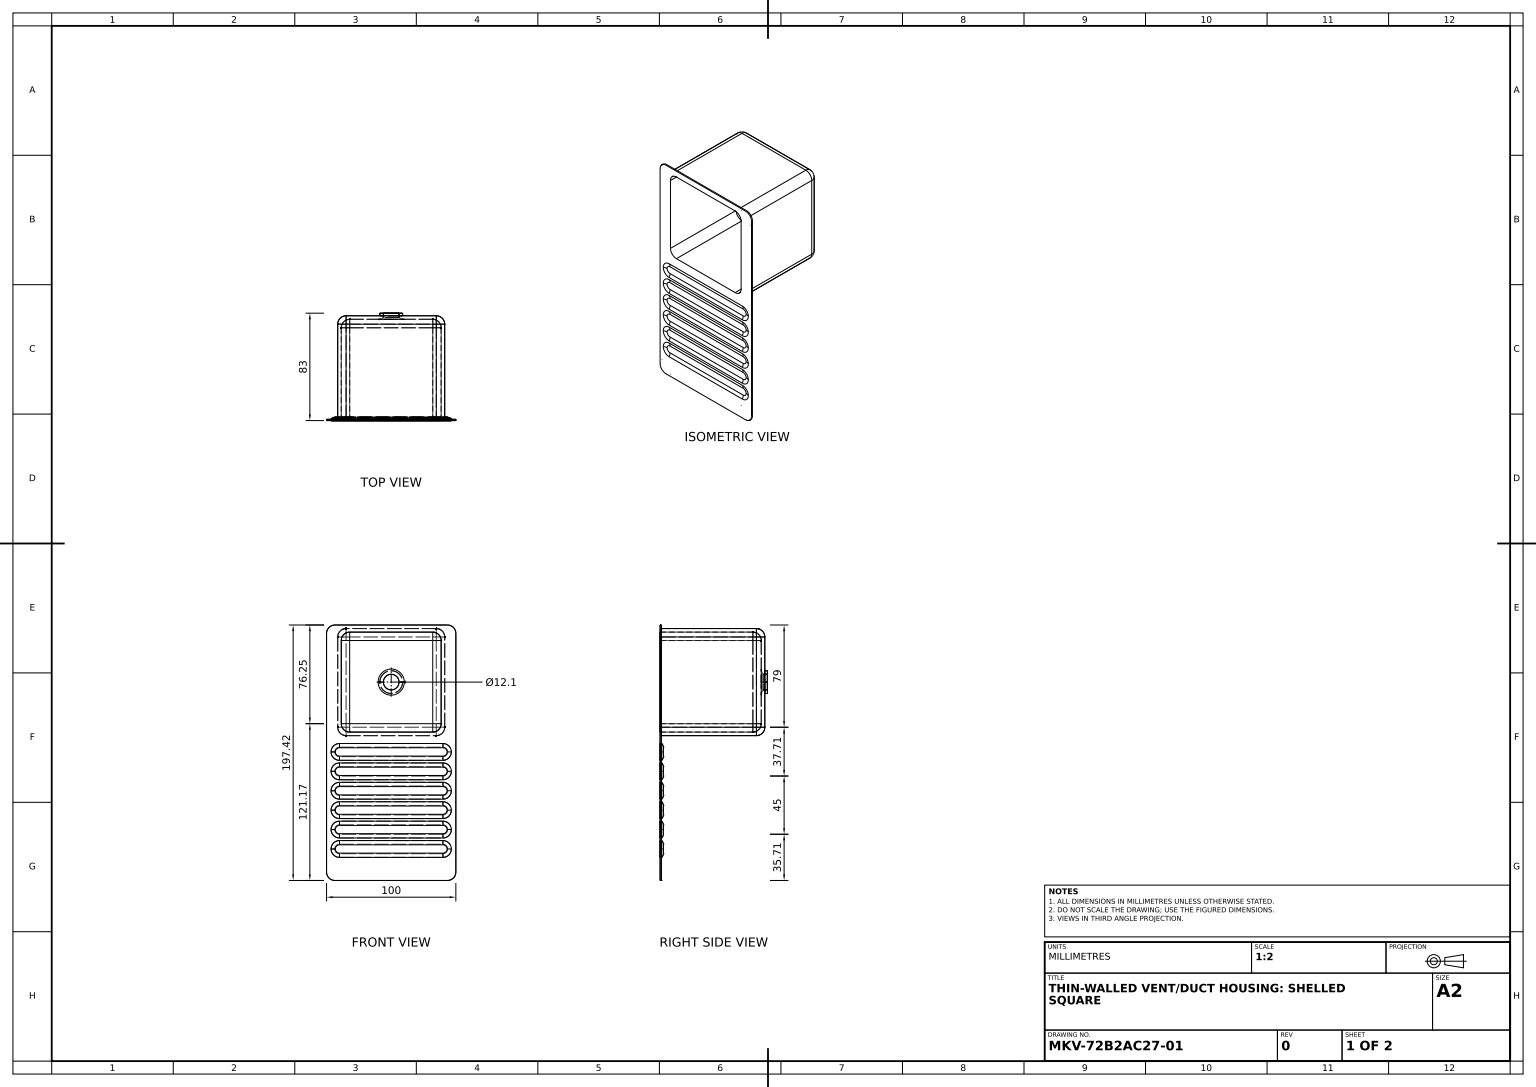
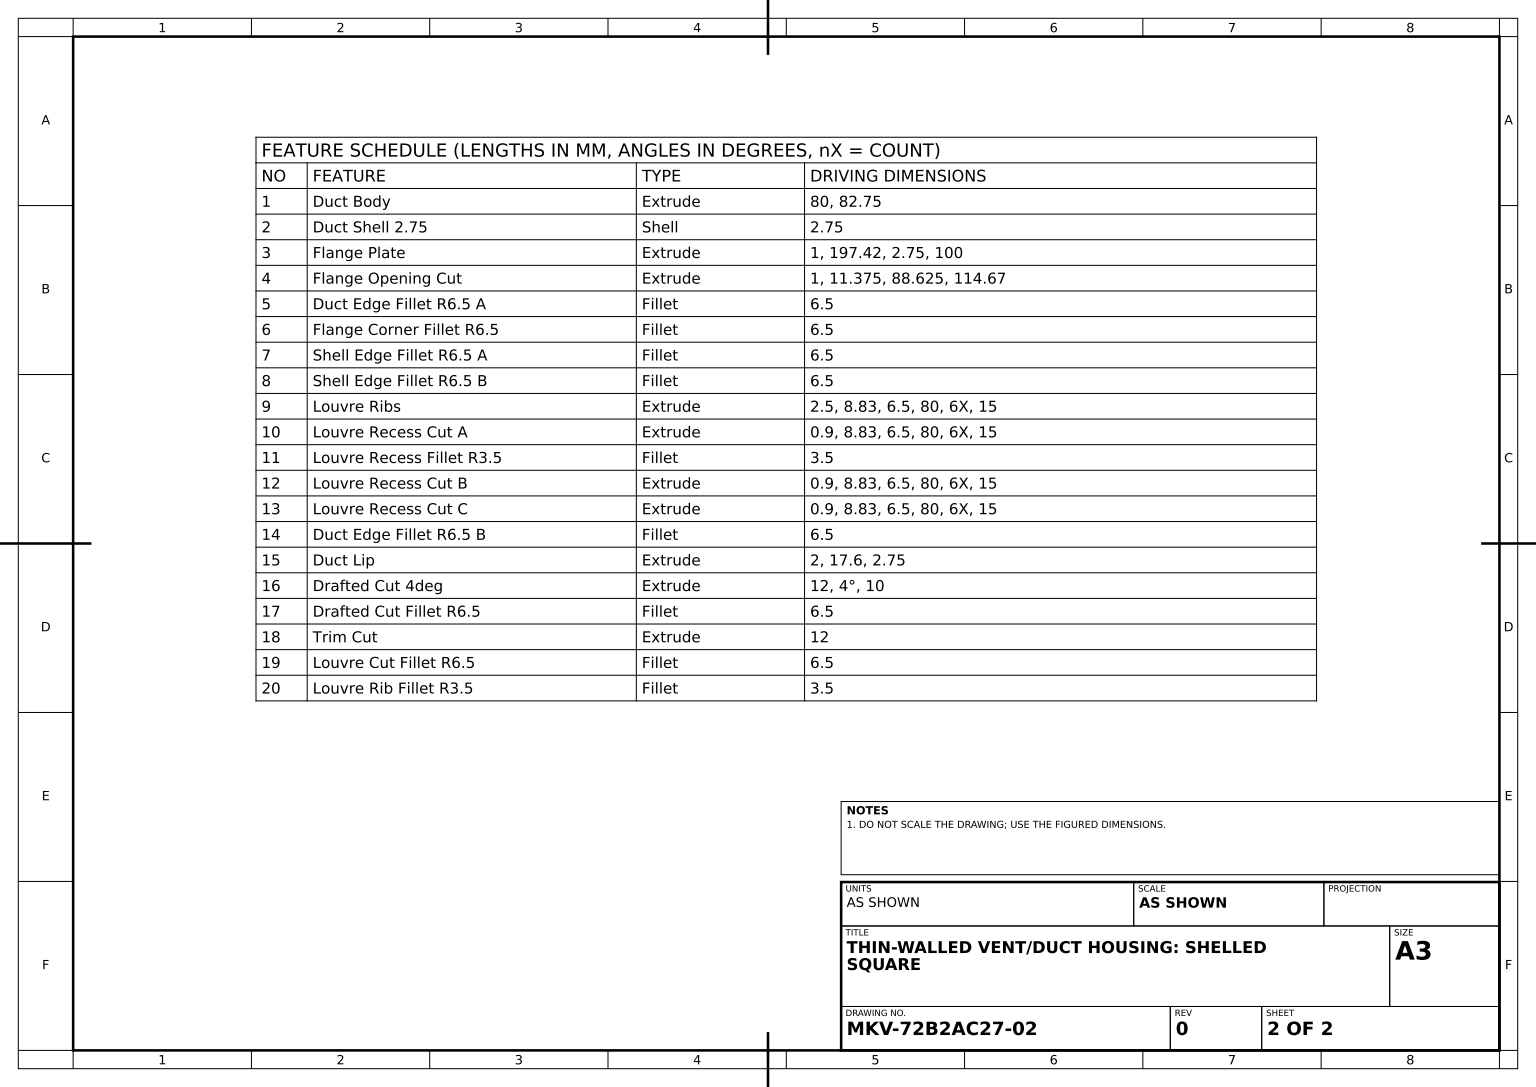
solid
v1 (40,-125.327281,38.5)
v2 (40,-132.582719,38.5)
e1 v1 v2 CIRCLE(AX(P(40,-128.955,38.5),D(0,0,-1),D(1,0,0)),3.627719)
v3 (-40,-132.582719,38.5)
e2 v2 v3 LINE
v4 (-43.627719,-128.955,38.5)
e3 v3 v4 CIRCLE(AX(P(-40,-128.955,38.5),D(0,0,-1),D(1,0,0)),3.627719)
v5 (-40,-125.327281,38.5)
e4 v4 v5 CIRCLE(AX(P(-40,-128.955,38.5),D(0,0,-1),D(1,0,0)),3.627719)
e5 v5 v1 LINE
face PLANE(AX(P(-40,-128.955,38.5),D(0,0,1),D(1,0,0))) rev [e1 e2 e3 e4 e5]
v6 (-40,-105.455,40)
v7 (40,-105.455,40)
e6 v6 v7 LINE
v8 (-40,-102.582719,38.5)
e7 v6 v8 CIRCLE(AX(P(-40,-102.582719,42),D(1,0,0),D(0,1,0)),3.5)
v9 (40,-102.582719,38.5)
e8 v9 v8 LINE
e9 v9 v7 CIRCLE(AX(P(40,-102.582719,42),D(-1,0,0),D(0,0,1)),3.5)
face CYL(AX(P(-40,-102.582719,42),D(-1,0,0),D(0,0,1)),3.5) [-e6 e7 -e8 e9]
v10 (-8.8,0,-42)
v11 (-8.8,0,-40)
e10 v10 v11 LINE
v12 (8.8,0,-42)
e11 v12 v10 CIRCLE(AX(P(0,0,-42),D(0,0,-1),D(-1,0,0)),8.8)
v13 (8.8,0,-40)
e12 v12 v13 LINE
e13 v13 v11 CIRCLE(AX(P(0,0,-40),D(0,0,-1),D(-1,0,0)),8.8)
face CYL(AX(P(0,0,-42),D(0,0,1),D(1,0,0)),8.8) [-e10 -e11 e12 e13]
v14 (-43.2,-53.955,40.1)
v15 (-40,-57.155,40.1)
e14 v14 v15 CIRCLE(AX(P(-40,-53.955,40.1),D(0,0,1),D(1,0,0)),3.2)
v16 (40,-57.155,40.1)
e15 v15 v16 LINE
v17 (43.2,-53.955,40.1)
e16 v16 v17 CIRCLE(AX(P(40,-53.955,40.1),D(0,0,1),D(1,0,0)),3.2)
v18 (40,-50.755,40.1)
e17 v17 v18 CIRCLE(AX(P(40,-53.955,40.1),D(0,0,1),D(1,0,0)),3.2)
v19 (-40,-50.755,40.1)
e18 v18 v19 LINE
e19 v19 v14 CIRCLE(AX(P(-40,-53.955,40.1),D(0,0,1),D(1,0,0)),3.2)
face PLANE(AX(P(-40,-53.955,40.1),D(0,0,1),D(1,0,0))) [e14 e15 e16 e17 e18 e19]
v20 (32.125,-32.125,-37.25)
v21 (32.125,32.125,-37.25)
e20 v20 v21 LINE
v22 (-32.125,32.125,-37.25)
e21 v21 v22 LINE
v23 (-32.125,-32.125,-37.25)
e22 v22 v23 LINE
e23 v23 v20 LINE
v24 (-10.116891,0,-37.25)
v25 (10.116891,0,-37.25)
e24 v24 v25 CIRCLE(AX(P(0,0,-37.25),D(0,0,-1),D(-1,0,0)),10.116891)
e25 v25 v24 CIRCLE(AX(P(0,0,-37.25),D(0,0,-1),D(-1,0,0)),10.116891)
face PLANE(AX(P(0,0,-37.25),D(0,0,-1),D(-1,0,0))) rev [e20 e21 e22 e23] [e24 e25]
v26 (-40,-122.455,40)
e26 v26 v5 CIRCLE(AX(P(-40,-125.327281,42),D(-1,0,0),D(0,0,1)),3.5)
v27 (40,-122.455,40)
e27 v27 v26 LINE
e28 v1 v27 CIRCLE(AX(P(40,-125.327281,42),D(1,0,0),D(0,0,-1)),3.5)
face CYL(AX(P(-40,-125.327281,42),D(1,0,0),D(0,1,0)),3.5) [-e5 -e26 -e27 -e28]
v28 (41.375,-34.875,-33.5)
v29 (41.375,34.875,-33.5)
e29 v28 v29 LINE
v30 (41.375,34.875,40)
e30 v29 v30 LINE
v31 (41.375,-34.875,40)
e31 v31 v30 LINE
e32 v31 v28 LINE
face PLANE(AX(P(41.375,-41.375,40),D(-1,0,0),D(0,0,1))) rev [e29 e30 -e31 e32]
v32 (40,-65.327281,38.5)
v33 (40,-72.582719,38.5)
e33 v32 v33 CIRCLE(AX(P(40,-68.955,38.5),D(0,0,-1),D(1,0,0)),3.627719)
v34 (-40,-72.582719,38.5)
e34 v33 v34 LINE
v35 (-43.627719,-68.955,38.5)
e35 v34 v35 CIRCLE(AX(P(-40,-68.955,38.5),D(0,0,-1),D(1,0,0)),3.627719)
v36 (-40,-65.327281,38.5)
e36 v35 v36 CIRCLE(AX(P(-40,-68.955,38.5),D(0,0,-1),D(1,0,0)),3.627719)
e37 v36 v32 LINE
face PLANE(AX(P(-40,-68.955,38.5),D(0,0,1),D(1,0,0))) rev [e33 e34 e35 e36 e37]
v37 (43.2,-68.955,40.1)
v38 (40,-65.755,40.1)
e38 v37 v38 CIRCLE(AX(P(40,-68.955,40.1),D(0,0,1),D(1,0,0)),3.2)
v39 (46.5,-68.955,41)
e39 v39 v37 CIRCLE(AX(P(43.2,-68.955,46.6),D(0,1,0),D(-1,0,0)),6.5)
v40 (40,-62.455,41)
e40 v39 v40 CIRCLE(AX(P(40,-68.955,41),D(0,0,1),D(1,0,0)),6.5)
e41 v38 v40 CIRCLE(AX(P(40,-65.755,46.6),D(1,0,0),D(0,0,-1)),6.5)
face TORUS(AX(P(40,-68.955,46.6),D(0,0,-1),D(-1,0,0)),3.2,6.5) rev [-e38 -e39 e40 -e41]
v41 (-38.625,32.125,-30.75)
v42 (-38.625,32.125,41)
e42 v41 v42 LINE
v43 (-32.125,38.625,-30.75)
e43 v41 v43 CIRCLE(AX(P(-32.125,32.125,-30.75),D(0,0,-1),D(1,0,0)),6.5)
v44 (-32.125,38.625,41)
e44 v44 v43 LINE
e45 v42 v44 CIRCLE(AX(P(-32.125,32.125,41),D(0,0,-1),D(1,0,0)),6.5)
face CYL(AX(P(-32.125,32.125,40),D(0,0,1),D(1,0,0)),6.5) rev [-e42 e43 -e44 -e45]
v45 (-6.05,0,-38.679458)
e46 v45 v24 CIRCLE(AX(P(-10.116891,0,-43.75),D(0,-1,0),D(0,0,-1)),6.5)
v46 (6.05,0,-38.679458)
e47 v46 v25 CIRCLE(AX(P(10.116891,0,-43.75),D(0,1,0),D(-1,0,0)),6.5)
e48 v45 v46 CIRCLE(AX(P(0,0,-38.679458),D(0,0,1),D(-1,0,0)),6.05)
face TORUS(AX(P(0,0,-43.75),D(0,0,-1),D(-1,0,0)),10.116891,6.5) [e46 -e25 -e47 -e48]
v47 (-46.5,-68.955,41)
v48 (-43.2,-68.955,40.1)
e49 v47 v48 CIRCLE(AX(P(-43.2,-68.955,46.6),D(0,-1,0),D(0,0,-1)),6.5)
v49 (-40,-75.455,41)
e50 v47 v49 CIRCLE(AX(P(-40,-68.955,41),D(0,0,1),D(1,0,0)),6.5)
v50 (-40,-72.155,40.1)
e51 v49 v50 CIRCLE(AX(P(-40,-72.155,46.6),D(1,0,0),D(0,0,-1)),6.5)
e52 v48 v50 CIRCLE(AX(P(-40,-68.955,40.1),D(0,0,1),D(1,0,0)),3.2)
face TORUS(AX(P(-40,-68.955,46.6),D(0,0,-1),D(-1,0,0)),3.2,6.5) rev [-e49 e50 e51 -e52]
v51 (-46.5,-113.955,40)
v52 (-43.627719,-113.955,38.5)
e53 v51 v52 CIRCLE(AX(P(-43.627719,-113.955,42),D(0,-1,0),D(0,0,-1)),3.5)
v53 (-40,-107.455,40)
e54 v53 v51 CIRCLE(AX(P(-40,-113.955,40),D(0,0,1),D(1,0,0)),6.5)
v54 (-40,-110.327281,38.5)
e55 v53 v54 CIRCLE(AX(P(-40,-110.327281,42),D(-1,0,0),D(0,0,1)),3.5)
e56 v52 v54 CIRCLE(AX(P(-40,-113.955,38.5),D(0,0,-1),D(1,0,0)),3.627719)
face TORUS(AX(P(-40,-113.955,42),D(0,0,-1),D(-1,0,0)),3.627719,3.5) [-e53 -e54 e55 -e56]
v55 (34.875,41.375,-33.5)
e57 v29 v55 CIRCLE(AX(P(34.875,34.875,-33.5),D(0,0,1),D(-1,0,0)),6.5)
v56 (34.875,41.375,40)
e58 v56 v55 LINE
e59 v30 v56 CIRCLE(AX(P(34.875,34.875,40),D(0,0,1),D(1,0,0)),6.5)
face CYL(AX(P(34.875,34.875,40),D(0,0,-1),D(-1,0,0)),6.5) [e57 -e58 -e59 -e30]
v57 (-40,-117.155,40.1)
v58 (40,-117.155,40.1)
e60 v57 v58 LINE
v59 (43.2,-113.955,40.1)
e61 v58 v59 CIRCLE(AX(P(40,-113.955,40.1),D(0,0,1),D(1,0,0)),3.2)
v60 (40,-110.755,40.1)
e62 v59 v60 CIRCLE(AX(P(40,-113.955,40.1),D(0,0,1),D(1,0,0)),3.2)
v61 (-40,-110.755,40.1)
e63 v60 v61 LINE
v62 (-43.2,-113.955,40.1)
e64 v61 v62 CIRCLE(AX(P(-40,-113.955,40.1),D(0,0,1),D(1,0,0)),3.2)
e65 v62 v57 CIRCLE(AX(P(-40,-113.955,40.1),D(0,0,1),D(1,0,0)),3.2)
face PLANE(AX(P(-40,-113.955,40.1),D(0,0,1),D(1,0,0))) [e60 e61 e62 e63 e64 e65]
v63 (40,-72.155,40.1)
e66 v63 v37 CIRCLE(AX(P(40,-68.955,40.1),D(0,0,1),D(1,0,0)),3.2)
v64 (40,-75.455,41)
e67 v63 v64 CIRCLE(AX(P(40,-72.155,46.6),D(-1,0,0),D(0,0,1)),6.5)
e68 v64 v39 CIRCLE(AX(P(40,-68.955,41),D(0,0,1),D(1,0,0)),6.5)
face TORUS(AX(P(40,-68.955,46.6),D(0,0,-1),D(-1,0,0)),3.2,6.5) rev [e39 -e66 e67 e68]
v65 (40,-135.455,40)
e69 v2 v65 CIRCLE(AX(P(40,-132.582719,42),D(-1,0,0),D(0,0,1)),3.5)
e70 v65 v27 CIRCLE(AX(P(40,-128.955,40),D(0,0,1),D(1,0,0)),6.5)
face TORUS(AX(P(40,-128.955,42),D(0,0,-1),D(-1,0,0)),3.627719,3.5) [-e69 -e1 e28 -e70]
v66 (-34.875,41.375,-33.5)
v67 (-34.875,34.875,-40)
e71 v66 v67 CIRCLE(AX(P(-34.875,34.875,-33.5),D(-1,0,0),D(0,0,1)),6.5)
v68 (-41.375,34.875,-33.5)
e72 v67 v68 CIRCLE(AX(P(-34.875,34.875,-33.5),D(0,1,0),D(0,0,1)),6.5)
e73 v66 v68 CIRCLE(AX(P(-34.875,34.875,-33.5),D(0,0,1),D(-1,0,0)),6.5)
face SPHERE(AX(P(-34.875,34.875,-33.5),D(0,1,0),D(-1,0,0)),6.5) [e71 e72 -e73]
v69 (40,-62.455,40)
e74 v32 v69 CIRCLE(AX(P(40,-65.327281,42),D(1,0,0),D(0,0,-1)),3.5)
v70 (40,-75.455,40)
e75 v70 v69 CIRCLE(AX(P(40,-68.955,40),D(0,0,1),D(1,0,0)),6.5)
e76 v33 v70 CIRCLE(AX(P(40,-72.582719,42),D(-1,0,0),D(0,0,1)),3.5)
face TORUS(AX(P(40,-68.955,42),D(0,0,-1),D(-1,0,0)),3.627719,3.5) [e74 -e75 -e76 -e33]
v71 (43.5,-153.295,41)
v72 (50,-146.795,41)
e77 v71 v72 CIRCLE(AX(P(43.5,-146.795,41),D(0,0,1),D(1,0,0)),6.5)
v73 (43.5,-153.295,40)
e78 v73 v71 LINE
v74 (50,-146.795,40)
e79 v74 v73 CIRCLE(AX(P(43.5,-146.795,40),D(0,0,-1),D(1,0,0)),6.5)
e80 v72 v74 LINE
face CYL(AX(P(43.5,-146.795,41),D(0,0,-1),D(-1,0,0)),6.5) [-e77 -e78 -e79 -e80]
v75 (40,-47.455,41)
e81 v18 v75 CIRCLE(AX(P(40,-50.755,46.6),D(1,0,0),D(0,0,-1)),6.5)
v76 (46.5,-53.955,41)
e82 v76 v17 CIRCLE(AX(P(43.2,-53.955,46.6),D(0,1,0),D(-1,0,0)),6.5)
e83 v76 v75 CIRCLE(AX(P(40,-53.955,41),D(0,0,1),D(1,0,0)),6.5)
face TORUS(AX(P(40,-53.955,46.6),D(0,0,-1),D(-1,0,0)),3.2,6.5) rev [-e81 -e17 -e82 e83]
e84 v11 v13 CIRCLE(AX(P(0,0,-40),D(0,0,-1),D(-1,0,0)),8.8)
e85 v10 v12 CIRCLE(AX(P(0,0,-42),D(0,0,-1),D(-1,0,0)),8.8)
face CYL(AX(P(0,0,-42),D(0,0,1),D(1,0,0)),8.8) [e84 -e12 -e85 e10]
v77 (-43.627719,-98.955,38.5)
v78 (-40,-95.327281,38.5)
e86 v77 v78 CIRCLE(AX(P(-40,-98.955,38.5),D(0,0,-1),D(1,0,0)),3.627719)
v79 (40,-95.327281,38.5)
e87 v78 v79 LINE
e88 v79 v9 CIRCLE(AX(P(40,-98.955,38.5),D(0,0,-1),D(1,0,0)),3.627719)
e89 v8 v77 CIRCLE(AX(P(-40,-98.955,38.5),D(0,0,-1),D(1,0,0)),3.627719)
face PLANE(AX(P(-40,-98.955,38.5),D(0,0,1),D(1,0,0))) rev [e86 e87 e88 e8 e89]
v80 (40,-87.155,40.1)
v81 (43.2,-83.955,40.1)
e90 v80 v81 CIRCLE(AX(P(40,-83.955,40.1),D(0,0,1),D(1,0,0)),3.2)
v82 (40,-90.455,41)
e91 v80 v82 CIRCLE(AX(P(40,-87.155,46.6),D(-1,0,0),D(0,0,1)),6.5)
v83 (46.5,-83.955,41)
e92 v82 v83 CIRCLE(AX(P(40,-83.955,41),D(0,0,1),D(1,0,0)),6.5)
e93 v83 v81 CIRCLE(AX(P(43.2,-83.955,46.6),D(0,1,0),D(-1,0,0)),6.5)
face TORUS(AX(P(40,-83.955,46.6),D(0,0,-1),D(-1,0,0)),3.2,6.5) rev [-e90 e91 e92 e93]
v84 (34.875,34.875,-40)
v85 (34.875,-34.875,-40)
e94 v84 v85 LINE
v86 (-34.875,-34.875,-40)
e95 v85 v86 LINE
e96 v86 v67 LINE
e97 v67 v84 LINE
face PLANE(AX(P(0,0,-40),D(0,0,-1),D(-1,0,0))) [-e84 -e13] [e94 e95 e96 e97]
v87 (-40,-105.455,41)
v88 (-40,-102.155,40.1)
e98 v87 v88 CIRCLE(AX(P(-40,-102.155,46.6),D(1,0,0),D(0,0,-1)),6.5)
v89 (-43.2,-98.955,40.1)
e99 v89 v88 CIRCLE(AX(P(-40,-98.955,40.1),D(0,0,1),D(1,0,0)),3.2)
v90 (-46.5,-98.955,41)
e100 v90 v89 CIRCLE(AX(P(-43.2,-98.955,46.6),D(0,-1,0),D(0,0,-1)),6.5)
e101 v90 v87 CIRCLE(AX(P(-40,-98.955,41),D(0,0,1),D(1,0,0)),6.5)
face TORUS(AX(P(-40,-98.955,46.6),D(0,0,-1),D(-1,0,0)),3.2,6.5) rev [e98 -e99 -e100 e101]
v91 (43.5,44.125,40)
v92 (50,37.625,40)
e102 v91 v92 CIRCLE(AX(P(43.5,37.625,40),D(0,0,-1),D(1,0,0)),6.5)
e103 v74 v92 LINE
v93 (-43.5,-153.295,40)
e104 v93 v73 LINE
v94 (-50,-146.795,40)
e105 v93 v94 CIRCLE(AX(P(-43.5,-146.795,40),D(0,0,-1),D(1,0,0)),6.5)
v95 (-50,37.625,40)
e106 v95 v94 LINE
v96 (-43.5,44.125,40)
e107 v95 v96 CIRCLE(AX(P(-43.5,37.625,40),D(0,0,-1),D(1,0,0)),6.5)
e108 v91 v96 LINE
v97 (-40,-60.455,40)
v98 (40,-60.455,40)
e109 v97 v98 LINE
v99 (40,-47.455,40)
e110 v98 v99 CIRCLE(AX(P(40,-53.955,40),D(0,0,1),D(1,0,0)),6.5)
v100 (-40,-47.455,40)
e111 v99 v100 LINE
v101 (-46.5,-53.955,40)
e112 v100 v101 CIRCLE(AX(P(-40,-53.955,40),D(0,0,1),D(1,0,0)),6.5)
e113 v101 v97 CIRCLE(AX(P(-40,-53.955,40),D(0,0,1),D(1,0,0)),6.5)
v102 (-46.5,-128.955,40)
e114 v26 v102 CIRCLE(AX(P(-40,-128.955,40),D(0,0,1),D(1,0,0)),6.5)
v103 (-40,-135.455,40)
e115 v102 v103 CIRCLE(AX(P(-40,-128.955,40),D(0,0,1),D(1,0,0)),6.5)
e116 v103 v65 LINE
v104 (40,-90.455,40)
v105 (40,-77.455,40)
e117 v104 v105 CIRCLE(AX(P(40,-83.955,40),D(0,0,1),D(1,0,0)),6.5)
v106 (-40,-77.455,40)
e118 v105 v106 LINE
v107 (-46.5,-83.955,40)
e119 v106 v107 CIRCLE(AX(P(-40,-83.955,40),D(0,0,1),D(1,0,0)),6.5)
v108 (-40,-90.455,40)
e120 v107 v108 CIRCLE(AX(P(-40,-83.955,40),D(0,0,1),D(1,0,0)),6.5)
e121 v108 v104 LINE
v109 (-40,-62.455,40)
e122 v69 v109 LINE
v110 (-46.5,-68.955,40)
e123 v109 v110 CIRCLE(AX(P(-40,-68.955,40),D(0,0,1),D(1,0,0)),6.5)
v111 (-40,-75.455,40)
e124 v110 v111 CIRCLE(AX(P(-40,-68.955,40),D(0,0,1),D(1,0,0)),6.5)
e125 v111 v70 LINE
v112 (40,-92.455,40)
v113 (-40,-92.455,40)
e126 v112 v113 LINE
v114 (-46.5,-98.955,40)
e127 v113 v114 CIRCLE(AX(P(-40,-98.955,40),D(0,0,1),D(1,0,0)),6.5)
e128 v114 v6 CIRCLE(AX(P(-40,-98.955,40),D(0,0,1),D(1,0,0)),6.5)
e129 v7 v112 CIRCLE(AX(P(40,-98.955,40),D(0,0,1),D(1,0,0)),6.5)
v115 (-41.375,-34.875,40)
v116 (-34.875,-41.375,40)
e130 v115 v116 CIRCLE(AX(P(-34.875,-34.875,40),D(0,0,1),D(1,0,0)),6.5)
v117 (34.875,-41.375,40)
e131 v116 v117 LINE
e132 v117 v31 CIRCLE(AX(P(34.875,-34.875,40),D(0,0,1),D(1,0,0)),6.5)
v118 (-34.875,41.375,40)
e133 v56 v118 LINE
v119 (-41.375,34.875,40)
e134 v118 v119 CIRCLE(AX(P(-34.875,34.875,40),D(0,0,1),D(1,0,0)),6.5)
e135 v119 v115 LINE
v120 (-40,-120.455,40)
v121 (40,-120.455,40)
e136 v120 v121 LINE
v122 (40,-107.455,40)
e137 v121 v122 CIRCLE(AX(P(40,-113.955,40),D(0,0,1),D(1,0,0)),6.5)
e138 v122 v53 LINE
e139 v51 v120 CIRCLE(AX(P(-40,-113.955,40),D(0,0,1),D(1,0,0)),6.5)
face PLANE(AX(P(0,0,40),D(0,0,1),D(1,0,0))) rev [e102 -e103 e79 -e104 e105 -e106 e107 -e108] [e109 e110 e111 e112 e113] [e27 e114 e115 e116 e70] [e117 e118 e119 e120 e121] [e75 e122 e123 e124 e125] [e126 e127 e128 e6 e129] [e130 e131 e132 e31 e59 e133 e134 e135] [e136 e137 e138 e54 e139]
v123 (-34.875,-41.375,-33.5)
v124 (34.875,-41.375,-33.5)
e140 v123 v124 LINE
e141 v124 v117 LINE
e142 v116 v123 LINE
face PLANE(AX(P(-41.375,-41.375,40),D(0,1,0),D(0,0,1))) rev [e140 e141 -e131 e142]
e143 v114 v77 CIRCLE(AX(P(-43.627719,-98.955,42),D(0,-1,0),D(0,0,-1)),3.5)
face TORUS(AX(P(-40,-98.955,42),D(0,0,-1),D(-1,0,0)),3.627719,3.5) [-e128 e143 -e89 -e7]
e144 v29 v84 CIRCLE(AX(P(34.875,34.875,-33.5),D(0,1,0),D(0,0,1)),6.5)
e145 v55 v84 CIRCLE(AX(P(34.875,34.875,-33.5),D(-1,0,0),D(0,0,1)),6.5)
face SPHERE(AX(P(34.875,34.875,-33.5),D(0,1,0),D(-1,0,0)),6.5) [e144 -e145 -e57]
v125 (-40,-50.327281,38.5)
v126 (40,-50.327281,38.5)
e146 v125 v126 LINE
e147 v100 v125 CIRCLE(AX(P(-40,-50.327281,42),D(-1,0,0),D(0,0,1)),3.5)
e148 v126 v99 CIRCLE(AX(P(40,-50.327281,42),D(1,0,0),D(0,0,-1)),3.5)
face CYL(AX(P(-40,-50.327281,42),D(1,0,0),D(0,1,0)),3.5) [-e146 -e147 -e111 -e148]
v127 (-40,-122.455,41)
v128 (-40,-125.755,40.1)
e149 v127 v128 CIRCLE(AX(P(-40,-125.755,46.6),D(-1,0,0),D(0,-1,0)),6.5)
v129 (-46.5,-128.955,41)
e150 v127 v129 CIRCLE(AX(P(-40,-128.955,41),D(0,0,1),D(1,0,0)),6.5)
v130 (-43.2,-128.955,40.1)
e151 v129 v130 CIRCLE(AX(P(-43.2,-128.955,46.6),D(0,-1,0),D(0,0,-1)),6.5)
e152 v128 v130 CIRCLE(AX(P(-40,-128.955,40.1),D(0,0,1),D(1,0,0)),3.2)
face TORUS(AX(P(-40,-128.955,46.6),D(0,0,-1),D(-1,0,0)),3.2,6.5) rev [-e149 e150 e151 -e152]
v131 (38.625,32.125,41)
v132 (38.625,32.125,-30.75)
e153 v131 v132 LINE
v133 (38.625,-32.125,-30.75)
e154 v132 v133 LINE
v134 (38.625,-32.125,41)
e155 v133 v134 LINE
e156 v134 v131 LINE
face PLANE(AX(P(38.625,-41.375,40),D(-1,0,0),D(0,0,1))) [e153 e154 e155 e156]
v135 (40,-135.455,41)
v136 (46.5,-128.955,41)
e157 v135 v136 CIRCLE(AX(P(40,-128.955,41),D(0,0,1),D(1,0,0)),6.5)
v137 (43.2,-128.955,40.1)
e158 v136 v137 CIRCLE(AX(P(43.2,-128.955,46.6),D(0,1,0),D(-1,0,0)),6.5)
v138 (40,-132.155,40.1)
e159 v138 v137 CIRCLE(AX(P(40,-128.955,40.1),D(0,0,1),D(1,0,0)),3.2)
e160 v138 v135 CIRCLE(AX(P(40,-132.155,46.6),D(-1,0,0),D(0,0,1)),6.5)
face TORUS(AX(P(40,-128.955,46.6),D(0,0,-1),D(-1,0,0)),3.2,6.5) rev [e157 e158 -e159 e160]
v139 (40,-77.455,41)
e161 v83 v139 CIRCLE(AX(P(40,-83.955,41),D(0,0,1),D(1,0,0)),6.5)
v140 (40,-80.755,40.1)
e162 v140 v139 CIRCLE(AX(P(40,-80.755,46.6),D(1,0,0),D(0,0,-1)),6.5)
e163 v81 v140 CIRCLE(AX(P(40,-83.955,40.1),D(0,0,1),D(1,0,0)),3.2)
face TORUS(AX(P(40,-83.955,46.6),D(0,0,-1),D(-1,0,0)),3.2,6.5) rev [e161 -e162 -e163 -e93]
v141 (40,-110.327281,38.5)
e164 v54 v141 LINE
v142 (40,-117.582719,38.5)
e165 v141 v142 CIRCLE(AX(P(40,-113.955,38.5),D(0,0,-1),D(1,0,0)),3.627719)
v143 (-40,-117.582719,38.5)
e166 v142 v143 LINE
e167 v143 v52 CIRCLE(AX(P(-40,-113.955,38.5),D(0,0,-1),D(1,0,0)),3.627719)
face PLANE(AX(P(-40,-113.955,38.5),D(0,0,1),D(1,0,0))) rev [e164 e165 e166 e167 e56]
e168 v46 v45 CIRCLE(AX(P(0,0,-38.679458),D(0,0,1),D(-1,0,0)),6.05)
face TORUS(AX(P(0,0,-43.75),D(0,0,-1),D(-1,0,0)),10.116891,6.5) [-e24 -e46 -e168 e47]
v144 (-32.125,-38.625,-30.75)
e169 v23 v144 CIRCLE(AX(P(-32.125,-32.125,-30.75),D(-1,0,0),D(0,0,1)),6.5)
v145 (32.125,-38.625,-30.75)
e170 v145 v144 LINE
e171 v20 v145 CIRCLE(AX(P(32.125,-32.125,-30.75),D(-1,0,0),D(0,0,1)),6.5)
face CYL(AX(P(0,-32.125,-30.75),D(1,0,0),D(0,0,-1)),6.5) rev [-e23 e169 -e170 -e171]
v146 (-40,-92.455,41)
e172 v146 v90 CIRCLE(AX(P(-40,-98.955,41),D(0,0,1),D(1,0,0)),6.5)
v147 (-40,-95.755,40.1)
e173 v147 v89 CIRCLE(AX(P(-40,-98.955,40.1),D(0,0,1),D(1,0,0)),3.2)
e174 v146 v147 CIRCLE(AX(P(-40,-95.755,46.6),D(-1,0,0),D(0,-1,0)),6.5)
face TORUS(AX(P(-40,-98.955,46.6),D(0,0,-1),D(-1,0,0)),3.2,6.5) rev [e172 e100 -e173 -e174]
v148 (-40,-62.455,41)
e175 v148 v40 LINE
v149 (-40,-65.755,40.1)
e176 v148 v149 CIRCLE(AX(P(-40,-65.755,46.6),D(-1,0,0),D(0,-1,0)),6.5)
e177 v38 v149 LINE
face CYL(AX(P(-40,-65.755,46.6),D(-1,0,0),D(0,-1,0)),6.5) rev [-e175 e176 -e177 e41]
v150 (40,-102.155,40.1)
v151 (40,-105.455,41)
e178 v150 v151 CIRCLE(AX(P(40,-102.155,46.6),D(-1,0,0),D(0,0,1)),6.5)
e179 v88 v150 LINE
e180 v87 v151 LINE
face CYL(AX(P(-40,-102.155,46.6),D(-1,0,0),D(0,0,1)),6.5) rev [-e178 -e179 -e98 e180]
v152 (-6.05,0,-42)
v153 (6.05,0,-42)
e181 v152 v153 CIRCLE(AX(P(0,0,-42),D(0,0,-1),D(-1,0,0)),6.05)
e182 v153 v152 CIRCLE(AX(P(0,0,-42),D(0,0,-1),D(-1,0,0)),6.05)
face PLANE(AX(P(0,0,-42),D(0,0,-1),D(-1,0,0))) [-e181 -e182] [e11 e85]
e183 v55 v66 LINE
e184 v66 v118 LINE
face PLANE(AX(P(-41.375,41.375,40),D(0,-1,0),D(0,0,-1))) rev [e183 e184 -e133 e58]
e185 v79 v112 CIRCLE(AX(P(40,-95.327281,42),D(1,0,0),D(0,0,-1)),3.5)
e186 v113 v78 CIRCLE(AX(P(-40,-95.327281,42),D(-1,0,0),D(0,0,1)),3.5)
face CYL(AX(P(-40,-95.327281,42),D(1,0,0),D(0,1,0)),3.5) [-e126 -e185 -e87 -e186]
v154 (40,-60.455,41)
e187 v16 v154 CIRCLE(AX(P(40,-57.155,46.6),D(-1,0,0),D(0,0,1)),6.5)
e188 v154 v76 CIRCLE(AX(P(40,-53.955,41),D(0,0,1),D(1,0,0)),6.5)
face TORUS(AX(P(40,-53.955,46.6),D(0,0,-1),D(-1,0,0)),3.2,6.5) rev [e187 e188 e82 -e16]
v155 (-40,-80.327281,38.5)
v156 (40,-80.327281,38.5)
e189 v155 v156 LINE
v157 (40,-87.582719,38.5)
e190 v156 v157 CIRCLE(AX(P(40,-83.955,38.5),D(0,0,-1),D(1,0,0)),3.627719)
v158 (-40,-87.582719,38.5)
e191 v157 v158 LINE
v159 (-43.627719,-83.955,38.5)
e192 v158 v159 CIRCLE(AX(P(-40,-83.955,38.5),D(0,0,-1),D(1,0,0)),3.627719)
e193 v159 v155 CIRCLE(AX(P(-40,-83.955,38.5),D(0,0,-1),D(1,0,0)),3.627719)
face PLANE(AX(P(-40,-83.955,38.5),D(0,0,1),D(1,0,0))) rev [e189 e190 e191 e192 e193]
e194 v120 v143 CIRCLE(AX(P(-40,-117.582719,42),D(1,0,0),D(0,1,0)),3.5)
face TORUS(AX(P(-40,-113.955,42),D(0,0,-1),D(-1,0,0)),3.627719,3.5) [-e194 -e139 e53 -e167]
v160 (-40,-47.455,41)
e195 v160 v19 CIRCLE(AX(P(-40,-50.755,46.6),D(-1,0,0),D(0,-1,0)),6.5)
v161 (-46.5,-53.955,41)
e196 v160 v161 CIRCLE(AX(P(-40,-53.955,41),D(0,0,1),D(1,0,0)),6.5)
e197 v161 v14 CIRCLE(AX(P(-43.2,-53.955,46.6),D(0,-1,0),D(0,0,-1)),6.5)
face TORUS(AX(P(-40,-53.955,46.6),D(0,0,-1),D(-1,0,0)),3.2,6.5) rev [-e195 e196 e197 -e19]
v162 (-41.375,-34.875,-33.5)
e198 v162 v123 CIRCLE(AX(P(-34.875,-34.875,-33.5),D(0,0,1),D(-1,0,0)),6.5)
e199 v86 v162 CIRCLE(AX(P(-34.875,-34.875,-33.5),D(0,1,0),D(0,0,1)),6.5)
e200 v86 v123 CIRCLE(AX(P(-34.875,-34.875,-33.5),D(-1,0,0),D(0,0,1)),6.5)
face SPHERE(AX(P(-34.875,-34.875,-33.5),D(0,1,0),D(-1,0,0)),6.5) [-e198 -e199 e200]
v163 (-40,-90.455,41)
v164 (-40,-87.155,40.1)
e201 v163 v164 CIRCLE(AX(P(-40,-87.155,46.6),D(1,0,0),D(0,0,-1)),6.5)
v165 (-43.2,-83.955,40.1)
e202 v165 v164 CIRCLE(AX(P(-40,-83.955,40.1),D(0,0,1),D(1,0,0)),3.2)
v166 (-46.5,-83.955,41)
e203 v166 v165 CIRCLE(AX(P(-43.2,-83.955,46.6),D(0,-1,0),D(0,0,-1)),6.5)
e204 v166 v163 CIRCLE(AX(P(-40,-83.955,41),D(0,0,1),D(1,0,0)),6.5)
face TORUS(AX(P(-40,-83.955,46.6),D(0,0,-1),D(-1,0,0)),3.2,6.5) rev [e201 -e202 -e203 e204]
v167 (-40,-120.455,41)
e205 v167 v57 CIRCLE(AX(P(-40,-117.155,46.6),D(1,0,0),D(0,0,-1)),6.5)
v168 (40,-120.455,41)
e206 v167 v168 LINE
e207 v58 v168 CIRCLE(AX(P(40,-117.155,46.6),D(-1,0,0),D(0,0,1)),6.5)
face CYL(AX(P(-40,-117.155,46.6),D(-1,0,0),D(0,-1,0)),6.5) rev [-e60 -e205 e206 -e207]
e208 v107 v159 CIRCLE(AX(P(-43.627719,-83.955,42),D(0,-1,0),D(0,0,-1)),3.5)
e209 v106 v155 CIRCLE(AX(P(-40,-80.327281,42),D(-1,0,0),D(0,0,1)),3.5)
face TORUS(AX(P(-40,-83.955,42),D(0,0,-1),D(-1,0,0)),3.627719,3.5) [-e193 -e208 -e119 e209]
v169 (-40,-77.455,41)
e210 v139 v169 LINE
v170 (-40,-80.755,40.1)
e211 v169 v170 CIRCLE(AX(P(-40,-80.755,46.6),D(-1,0,0),D(0,-1,0)),6.5)
e212 v140 v170 LINE
face CYL(AX(P(-40,-80.755,46.6),D(1,0,0),D(0,0,-1)),6.5) rev [e210 e211 -e212 e162]
v171 (40,-107.455,41)
e213 v60 v171 CIRCLE(AX(P(40,-110.755,46.6),D(1,0,0),D(0,0,-1)),6.5)
v172 (-40,-107.455,41)
e214 v171 v172 LINE
e215 v172 v61 CIRCLE(AX(P(-40,-110.755,46.6),D(-1,0,0),D(0,-1,0)),6.5)
face CYL(AX(P(-40,-110.755,46.6),D(1,0,0),D(0,0,-1)),6.5) rev [e213 e214 e215 -e63]
v173 (40,-125.755,40.1)
e216 v173 v128 LINE
v174 (40,-122.455,41)
e217 v173 v174 CIRCLE(AX(P(40,-125.755,46.6),D(1,0,0),D(0,0,-1)),6.5)
e218 v174 v127 LINE
face CYL(AX(P(-40,-125.755,46.6),D(1,0,0),D(0,1,0)),6.5) rev [e149 -e216 e217 e218]
v175 (-43.627719,-53.955,38.5)
e219 v175 v125 CIRCLE(AX(P(-40,-53.955,38.5),D(0,0,-1),D(1,0,0)),3.627719)
e220 v101 v175 CIRCLE(AX(P(-43.627719,-53.955,42),D(0,-1,0),D(0,0,-1)),3.5)
face TORUS(AX(P(-40,-53.955,42),D(0,0,-1),D(-1,0,0)),3.627719,3.5) [-e112 e147 -e219 -e220]
v176 (-40,-60.455,41)
e221 v176 v15 CIRCLE(AX(P(-40,-57.155,46.6),D(1,0,0),D(0,0,-1)),6.5)
e222 v161 v176 CIRCLE(AX(P(-40,-53.955,41),D(0,0,1),D(1,0,0)),6.5)
face TORUS(AX(P(-40,-53.955,46.6),D(0,0,-1),D(-1,0,0)),3.2,6.5) rev [e221 -e14 -e197 e222]
v177 (-38.625,-32.125,-30.75)
e223 v144 v177 CIRCLE(AX(P(-32.125,-32.125,-30.75),D(0,0,-1),D(1,0,0)),6.5)
e224 v23 v177 CIRCLE(AX(P(-32.125,-32.125,-30.75),D(0,1,0),D(0,0,1)),6.5)
face SPHERE(AX(P(-32.125,-32.125,-30.75),D(0,1,0),D(-1,0,0)),6.5) rev [-e223 -e169 e224]
e225 v85 v124 CIRCLE(AX(P(34.875,-34.875,-33.5),D(-1,0,0),D(0,-1,0)),6.5)
face CYL(AX(P(-41.375,-34.875,-33.5),D(-1,0,0),D(0,0,1)),6.5) [-e200 -e95 e225 -e140]
e226 v111 v34 CIRCLE(AX(P(-40,-72.582719,42),D(1,0,0),D(0,1,0)),3.5)
face CYL(AX(P(-40,-72.582719,42),D(-1,0,0),D(0,0,1)),3.5) [-e34 e76 -e125 e226]
e227 v149 v48 CIRCLE(AX(P(-40,-68.955,40.1),D(0,0,1),D(1,0,0)),3.2)
e228 v50 v63 LINE
face PLANE(AX(P(-40,-68.955,40.1),D(0,0,1),D(1,0,0))) [e177 e227 e52 e228 e66 e38]
v178 (32.125,38.625,41)
e229 v178 v44 LINE
v179 (32.125,38.625,-30.75)
e230 v43 v179 LINE
e231 v179 v178 LINE
face PLANE(AX(P(-41.375,38.625,40),D(0,-1,0),D(0,0,-1))) [e229 e44 e230 e231]
v180 (-40,-132.155,40.1)
e232 v180 v138 LINE
v181 (-40,-135.455,41)
e233 v181 v180 CIRCLE(AX(P(-40,-132.155,46.6),D(1,0,0),D(0,0,-1)),6.5)
e234 v181 v135 LINE
face CYL(AX(P(-40,-132.155,46.6),D(-1,0,0),D(0,0,1)),6.5) rev [-e160 -e232 -e233 e234]
v182 (-40,-57.582719,38.5)
e235 v182 v175 CIRCLE(AX(P(-40,-53.955,38.5),D(0,0,-1),D(1,0,0)),3.627719)
e236 v97 v182 CIRCLE(AX(P(-40,-57.582719,42),D(1,0,0),D(0,1,0)),3.5)
face TORUS(AX(P(-40,-53.955,42),D(0,0,-1),D(-1,0,0)),3.627719,3.5) [-e113 e220 -e235 -e236]
e237 v68 v162 LINE
e238 v162 v115 LINE
e239 v119 v68 LINE
face PLANE(AX(P(-41.375,-41.375,40),D(1,0,0),D(0,0,-1))) rev [e237 e238 -e135 e239]
e240 v22 v41 CIRCLE(AX(P(-32.125,32.125,-30.75),D(0,1,0),D(0,0,1)),6.5)
e241 v177 v41 LINE
face CYL(AX(P(-32.125,0,-30.75),D(0,-1,0),D(0,0,-1)),6.5) rev [-e22 e240 -e241 -e224]
e242 v133 v145 CIRCLE(AX(P(32.125,-32.125,-30.75),D(0,0,-1),D(1,0,0)),6.5)
v183 (32.125,-38.625,41)
e243 v183 v145 LINE
e244 v134 v183 CIRCLE(AX(P(32.125,-32.125,41),D(0,0,-1),D(1,0,0)),6.5)
face CYL(AX(P(32.125,-32.125,40),D(0,0,1),D(1,0,0)),6.5) rev [-e155 e242 -e243 -e244]
face CYL(AX(P(-34.875,-34.875,40),D(0,0,-1),D(-1,0,0)),6.5) [-e238 e198 -e142 -e130]
e245 v148 v47 CIRCLE(AX(P(-40,-68.955,41),D(0,0,1),D(1,0,0)),6.5)
face TORUS(AX(P(-40,-68.955,46.6),D(0,0,-1),D(-1,0,0)),3.2,6.5) rev [-e227 -e176 e245 e49]
e246 v109 v36 CIRCLE(AX(P(-40,-65.327281,42),D(-1,0,0),D(0,0,1)),3.5)
e247 v110 v35 CIRCLE(AX(P(-43.627719,-68.955,42),D(0,-1,0),D(0,0,-1)),3.5)
face TORUS(AX(P(-40,-68.955,42),D(0,0,-1),D(-1,0,0)),3.627719,3.5) [-e123 e246 -e36 -e247]
e248 v179 v21 CIRCLE(AX(P(32.125,32.125,-30.75),D(-1,0,0),D(0,0,1)),6.5)
e249 v43 v22 CIRCLE(AX(P(-32.125,32.125,-30.75),D(-1,0,0),D(0,0,1)),6.5)
face CYL(AX(P(0,32.125,-30.75),D(-1,0,0),D(0,0,1)),6.5) rev [-e21 -e248 -e230 e249]
v184 (40,-92.455,41)
e250 v184 v146 LINE
v185 (46.5,-98.955,41)
e251 v185 v184 CIRCLE(AX(P(40,-98.955,41),D(0,0,1),D(1,0,0)),6.5)
e252 v151 v185 CIRCLE(AX(P(40,-98.955,41),D(0,0,1),D(1,0,0)),6.5)
e253 v136 v174 CIRCLE(AX(P(40,-128.955,41),D(0,0,1),D(1,0,0)),6.5)
e254 v129 v181 CIRCLE(AX(P(-40,-128.955,41),D(0,0,1),D(1,0,0)),6.5)
e255 v176 v154 LINE
e256 v160 v75 LINE
e257 v49 v64 LINE
v186 (46.5,-113.955,41)
e258 v168 v186 CIRCLE(AX(P(40,-113.955,41),D(0,0,1),D(1,0,0)),6.5)
v187 (-46.5,-113.955,41)
e259 v187 v167 CIRCLE(AX(P(-40,-113.955,41),D(0,0,1),D(1,0,0)),6.5)
e260 v172 v187 CIRCLE(AX(P(-40,-113.955,41),D(0,0,1),D(1,0,0)),6.5)
e261 v186 v171 CIRCLE(AX(P(40,-113.955,41),D(0,0,1),D(1,0,0)),6.5)
e262 v169 v166 CIRCLE(AX(P(-40,-83.955,41),D(0,0,1),D(1,0,0)),6.5)
e263 v163 v82 LINE
v188 (-32.125,-38.625,41)
e264 v188 v183 LINE
v189 (-38.625,-32.125,41)
e265 v188 v189 CIRCLE(AX(P(-32.125,-32.125,41),D(0,0,-1),D(1,0,0)),6.5)
e266 v42 v189 LINE
e267 v178 v131 CIRCLE(AX(P(32.125,32.125,41),D(0,0,-1),D(1,0,0)),6.5)
v190 (50,37.625,41)
e268 v72 v190 LINE
v191 (43.5,44.125,41)
e269 v190 v191 CIRCLE(AX(P(43.5,37.625,41),D(0,0,1),D(1,0,0)),6.5)
v192 (-43.5,44.125,41)
e270 v191 v192 LINE
v193 (-50,37.625,41)
e271 v192 v193 CIRCLE(AX(P(-43.5,37.625,41),D(0,0,1),D(1,0,0)),6.5)
v194 (-50,-146.795,41)
e272 v193 v194 LINE
v195 (-43.5,-153.295,41)
e273 v194 v195 CIRCLE(AX(P(-43.5,-146.795,41),D(0,0,1),D(1,0,0)),6.5)
e274 v195 v71 LINE
face PLANE(AX(P(0,0,41),D(0,0,1),D(1,0,0))) [-e250 -e251 -e252 -e180 -e101 -e172] [-e218 -e253 -e157 -e234 -e254 -e150] [-e255 -e222 -e196 e256 -e83 -e188] [-e245 e175 -e40 -e68 -e257 -e50] [-e258 -e206 -e259 -e260 -e214 -e261] [-e262 -e210 -e161 -e92 -e263 -e204] [e244 -e264 e265 -e266 e45 -e229 e267 -e156] [e268 e269 e270 e271 e272 e273 e274 e77]
e275 v92 v190 LINE
face PLANE(AX(P(50,44.125,41),D(-1,0,0),D(0,-1,0))) rev [e80 e103 e275 -e268]
e276 v28 v85 CIRCLE(AX(P(34.875,-34.875,-33.5),D(0,1,0),D(0,0,1)),6.5)
face CYL(AX(P(34.875,-41.375,-33.5),D(0,-1,0),D(0,0,-1)),6.5) [-e144 -e29 e276 -e94]
e277 v102 v4 CIRCLE(AX(P(-43.627719,-128.955,42),D(0,-1,0),D(0,0,-1)),3.5)
face TORUS(AX(P(-40,-128.955,42),D(0,0,-1),D(-1,0,0)),3.627719,3.5) [-e114 e26 -e4 -e277]
v196 (43.2,-98.955,40.1)
e278 v150 v196 CIRCLE(AX(P(40,-98.955,40.1),D(0,0,1),D(1,0,0)),3.2)
v197 (40,-95.755,40.1)
e279 v196 v197 CIRCLE(AX(P(40,-98.955,40.1),D(0,0,1),D(1,0,0)),3.2)
e280 v197 v147 LINE
face PLANE(AX(P(-40,-98.955,40.1),D(0,0,1),D(1,0,0))) [e278 e279 e280 e173 e99 e179]
e281 v130 v180 CIRCLE(AX(P(-40,-128.955,40.1),D(0,0,1),D(1,0,0)),3.2)
face TORUS(AX(P(-40,-128.955,46.6),D(0,0,-1),D(-1,0,0)),3.2,6.5) rev [e254 e233 -e281 -e151]
e282 v157 v104 CIRCLE(AX(P(40,-87.582719,42),D(-1,0,0),D(0,0,1)),3.5)
e283 v108 v158 CIRCLE(AX(P(-40,-87.582719,42),D(1,0,0),D(0,1,0)),3.5)
face CYL(AX(P(-40,-87.582719,42),D(-1,0,0),D(0,-1,0)),3.5) [-e191 e282 -e121 e283]
e284 v191 v91 LINE
e285 v96 v192 LINE
face PLANE(AX(P(-50,44.125,41),D(0,-1,0),D(1,0,0))) rev [e284 e108 e285 -e270]
e286 v156 v105 CIRCLE(AX(P(40,-80.327281,42),D(1,0,0),D(0,0,-1)),3.5)
face CYL(AX(P(-40,-80.327281,42),D(1,0,0),D(0,0,-1)),3.5) [-e118 -e286 -e189 -e209]
e287 v124 v28 CIRCLE(AX(P(34.875,-34.875,-33.5),D(0,0,1),D(-1,0,0)),6.5)
face SPHERE(AX(P(34.875,-34.875,-33.5),D(0,1,0),D(-1,0,0)),6.5) [-e287 -e225 -e276]
face CYL(AX(P(-34.875,-41.375,-33.5),D(0,1,0),D(0,0,1)),6.5) [-e96 e199 -e237 -e72]
e288 v189 v177 LINE
face PLANE(AX(P(-38.625,-41.375,40),D(1,0,0),D(0,0,-1))) [e42 e266 e288 e241]
e289 v195 v93 LINE
face PLANE(AX(P(-50,-153.295,41),D(0,1,0),D(0,0,1))) rev [e78 -e274 e289 e104]
e290 v137 v173 CIRCLE(AX(P(40,-128.955,40.1),D(0,0,1),D(1,0,0)),3.2)
face TORUS(AX(P(40,-128.955,46.6),D(0,0,-1),D(-1,0,0)),3.2,6.5) rev [-e217 -e290 -e158 e253]
e291 v103 v3 CIRCLE(AX(P(-40,-132.582719,42),D(1,0,0),D(0,1,0)),3.5)
face CYL(AX(P(-40,-132.582719,42),D(-1,0,0),D(0,0,1)),3.5) [e69 -e116 e291 -e2]
e292 v185 v196 CIRCLE(AX(P(43.2,-98.955,46.6),D(0,1,0),D(-1,0,0)),6.5)
face TORUS(AX(P(40,-98.955,46.6),D(0,0,-1),D(-1,0,0)),3.2,6.5) rev [-e278 e178 e252 e292]
e293 v144 v188 LINE
face PLANE(AX(P(-41.375,-38.625,40),D(0,1,0),D(0,0,1))) [e243 e170 e293 e264]
e294 v193 v95 LINE
face CYL(AX(P(-43.5,37.625,41),D(0,0,-1),D(-1,0,0)),6.5) [-e294 -e271 -e285 -e107]
v198 (40,-57.582719,38.5)
e295 v198 v182 LINE
e296 v198 v98 CIRCLE(AX(P(40,-57.582719,42),D(-1,0,0),D(0,0,1)),3.5)
face CYL(AX(P(-40,-57.582719,42),D(-1,0,0),D(0,-1,0)),3.5) [-e109 e236 -e295 e296]
face TORUS(AX(P(40,-83.955,42),D(0,0,-1),D(-1,0,0)),3.627719,3.5) [-e190 e286 -e117 -e282]
face TORUS(AX(P(-40,-98.955,42),D(0,0,-1),D(-1,0,0)),3.627719,3.5) [-e143 -e127 e186 -e86]
face TORUS(AX(P(-40,-83.955,42),D(0,0,-1),D(-1,0,0)),3.627719,3.5) [-e283 -e120 e208 -e192]
e297 v170 v165 CIRCLE(AX(P(-40,-83.955,40.1),D(0,0,1),D(1,0,0)),3.2)
e298 v164 v80 LINE
face PLANE(AX(P(-40,-83.955,40.1),D(0,0,1),D(1,0,0))) [e90 e163 e212 e297 e202 e298]
e299 v133 v20 CIRCLE(AX(P(32.125,-32.125,-30.75),D(0,1,0),D(0,0,1)),6.5)
face SPHERE(AX(P(32.125,-32.125,-30.75),D(0,1,0),D(-1,0,0)),6.5) rev [e299 e171 -e242]
face CYL(AX(P(34.875,-34.875,40),D(0,0,-1),D(-1,0,0)),6.5) [-e141 e287 -e32 -e132]
face TORUS(AX(P(-40,-83.955,46.6),D(0,0,-1),D(-1,0,0)),3.2,6.5) rev [-e297 -e211 e262 e203]
e300 v186 v59 CIRCLE(AX(P(43.2,-113.955,46.6),D(0,1,0),D(-1,0,0)),6.5)
face TORUS(AX(P(40,-113.955,46.6),D(0,0,-1),D(-1,0,0)),3.2,6.5) rev [e261 -e213 -e62 -e300]
e301 v141 v122 CIRCLE(AX(P(40,-110.327281,42),D(1,0,0),D(0,0,-1)),3.5)
face CYL(AX(P(-40,-110.327281,42),D(1,0,0),D(0,0,-1)),3.5) [-e55 -e138 -e301 -e164]
face CYL(AX(P(-40,-57.155,46.6),D(-1,0,0),D(0,-1,0)),6.5) rev [-e221 e255 -e187 -e15]
face CYL(AX(P(-34.875,34.875,40),D(0,0,-1),D(-1,0,0)),6.5) [e73 -e239 -e134 -e184]
face TORUS(AX(P(-40,-128.955,42),D(0,0,-1),D(-1,0,0)),3.627719,3.5) [-e3 -e291 -e115 e277]
e302 v132 v21 CIRCLE(AX(P(32.125,32.125,-30.75),D(0,1,0),D(0,0,1)),6.5)
face CYL(AX(P(32.125,0,-30.75),D(0,1,0),D(0,0,1)),6.5) rev [-e20 -e299 -e154 e302]
e303 v142 v121 CIRCLE(AX(P(40,-117.582719,42),D(-1,0,0),D(0,0,1)),3.5)
face CYL(AX(P(-40,-117.582719,42),D(-1,0,0),D(0,-1,0)),3.5) [e303 -e136 e194 -e166]
face TORUS(AX(P(-40,-68.955,42),D(0,0,-1),D(-1,0,0)),3.627719,3.5) [-e124 e247 -e35 -e226]
e304 v94 v194 LINE
face CYL(AX(P(-43.5,-146.795,41),D(0,0,-1),D(-1,0,0)),6.5) [-e304 -e105 -e289 -e273]
face TORUS(AX(P(40,-113.955,42),D(0,0,-1),D(-1,0,0)),3.627719,3.5) [e301 -e137 -e303 -e165]
face SPHERE(AX(P(-32.125,32.125,-30.75),D(0,1,0),D(-1,0,0)),6.5) rev [-e240 -e249 -e43]
e305 v187 v62 CIRCLE(AX(P(-43.2,-113.955,46.6),D(0,-1,0),D(0,0,-1)),6.5)
face TORUS(AX(P(-40,-113.955,46.6),D(0,0,-1),D(-1,0,0)),3.2,6.5) rev [e305 -e64 -e215 e260]
face CYL(AX(P(-41.375,34.875,-33.5),D(1,0,0),D(0,0,-1)),6.5) [-e71 -e183 e145 -e97]
face CYL(AX(P(-40,-87.155,46.6),D(-1,0,0),D(0,-1,0)),6.5) rev [-e298 -e201 e263 -e91]
face CYL(AX(P(-40,-72.155,46.6),D(-1,0,0),D(0,0,1)),6.5) rev [-e67 -e228 -e51 e257]
e306 v197 v184 CIRCLE(AX(P(40,-95.755,46.6),D(1,0,0),D(0,0,-1)),6.5)
face TORUS(AX(P(40,-98.955,46.6),D(0,0,-1),D(-1,0,0)),3.2,6.5) rev [e251 -e306 -e279 -e292]
face TORUS(AX(P(40,-113.955,46.6),D(0,0,-1),D(-1,0,0)),3.2,6.5) rev [e258 e300 -e61 e207]
face CYL(AX(P(43.5,37.625,41),D(0,0,-1),D(-1,0,0)),6.5) [-e102 -e284 -e269 -e275]
e307 v126 v198 CIRCLE(AX(P(40,-53.955,38.5),D(0,0,-1),D(1,0,0)),3.627719)
face TORUS(AX(P(40,-53.955,42),D(0,0,-1),D(-1,0,0)),3.627719,3.5) [-e110 -e296 -e307 e148]
face PLANE(AX(P(-40,-53.955,38.5),D(0,0,1),D(1,0,0))) rev [e295 e235 e219 e146 e307]
e308 v179 v132 CIRCLE(AX(P(32.125,32.125,-30.75),D(0,0,-1),D(1,0,0)),6.5)
face SPHERE(AX(P(32.125,32.125,-30.75),D(0,1,0),D(-1,0,0)),6.5) rev [e248 -e302 -e308]
face CYL(AX(P(-40,-95.755,46.6),D(1,0,0),D(0,1,0)),6.5) rev [e174 -e280 e306 e250]
face CYL(AX(P(32.125,32.125,40),D(0,0,1),D(1,0,0)),6.5) rev [e308 -e153 -e267 -e231]
face TORUS(AX(P(40,-98.955,42),D(0,0,-1),D(-1,0,0)),3.627719,3.5) [-e129 -e9 -e88 e185]
face CYL(AX(P(-40,-50.755,46.6),D(1,0,0),D(0,1,0)),6.5) rev [e81 -e256 e195 -e18]
face CYL(AX(P(-40,-65.327281,42),D(1,0,0),D(0,1,0)),3.5) [-e74 -e37 -e246 -e122]
face TORUS(AX(P(-40,-113.955,46.6),D(0,0,-1),D(-1,0,0)),3.2,6.5) rev [e205 -e65 -e305 e259]
face PLANE(AX(P(-40,-128.955,40.1),D(0,0,1),D(1,0,0))) [e232 e159 e290 e216 e152 e281]
e309 v152 v45 LINE
e310 v153 v46 LINE
face CYL(AX(P(0,0,-42),D(0,0,1),D(1,0,0)),6.05) rev [e309 e48 -e310 e182]
face PLANE(AX(P(-50,44.125,41),D(1,0,0),D(0,1,0))) rev [-e272 e294 e106 e304]
face CYL(AX(P(-32.125,-32.125,40),D(0,0,1),D(1,0,0)),6.5) rev [-e265 -e293 e223 -e288]
face CYL(AX(P(0,0,-42),D(0,0,1),D(1,0,0)),6.05) rev [e168 -e309 e181 e310]
